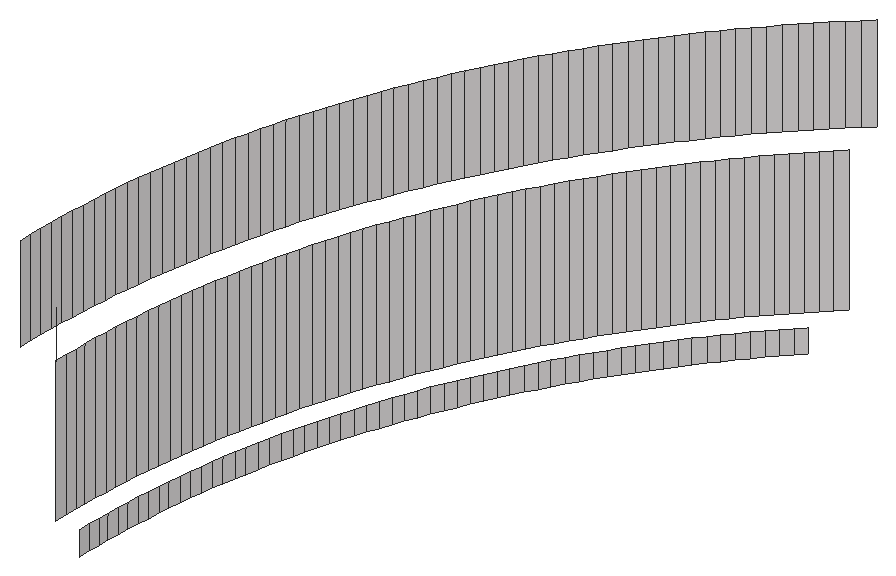
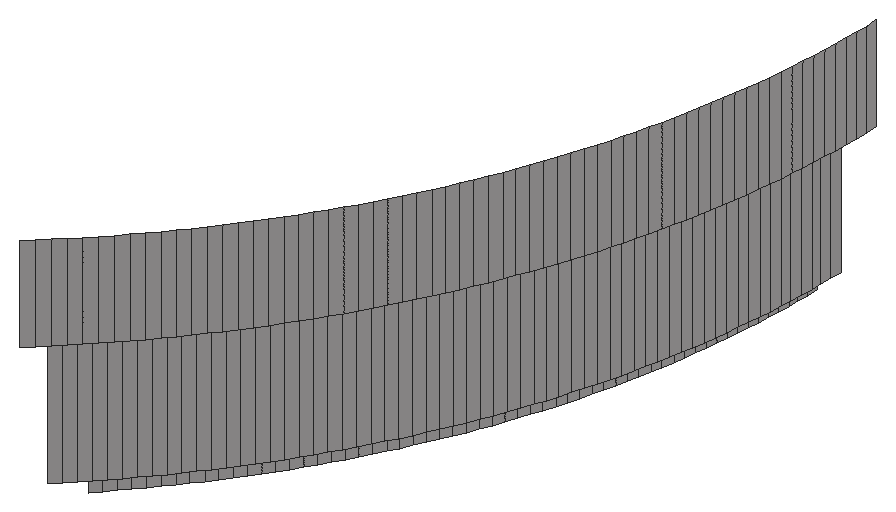
# SketchUp Ruby script. Lengths in inches.
U = 1.inch
M = Sketchup.active_model
def pt(a) = Geom::Point3d.new(a.map { |v| v * U })
def face(e, loops, mat)
  f = e.add_face(loops[0].map { |a| pt(a) })
  loops[1..].each { |l| e.add_face(l.map { |a| pt(a) }).erase! }
  f.material = f.back_material = mat if mat
  f
end
# faces: each face lists its corners as indices into pts; further lists are holes
def faces(e, pts, list, mat = nil) = list.each { |f| face(e, (f[0].is_a?(Array) ? f : [f]).map { |l| l.map { |i| pts[i] } }, mat) }
# xy, xz, yz: faces in a plane at the given z, y or x. An outline is a flat list of corners, or four numbers for a rectangle; further outlines are holes
def ring(l) = l.size == 4 ? [[l[0], l[1]], [l[2], l[1]], [l[2], l[3]], [l[0], l[3]]] : l.each_slice(2).to_a
def flat(e, list, mat, &to3) = list.each { |f| face(e, (f[0].is_a?(Array) ? f : [f]).map { |l| ring(l).map { |u, v| to3.(u, v) } }, mat) }
def xy(e, z, list, mat = nil) = flat(e, list, mat) { |x, y| [x, y, z] }
def xz(e, y, list, mat = nil) = flat(e, list, mat) { |x, z| [x, y, z] }
def yz(e, x, list, mat = nil) = flat(e, list, mat) { |y, z| [x, y, z] }
def lines(e, pts, list) = list.each { |a, b| e.add_line(pt(pts[a]), pt(pts[b])) }
# prism: a flat outline (further loops are holes) pulled along v
def prism(e, loops, v, mat = nil)
  f = face(e, loops, mat); d = Geom::Vector3d.new(v.map { |x| x * U })
  f.pushpull(f.normal.samedirection?(d) ? d.length : -d.length)
end
def box(e, o, s, mat = nil) = prism(e, [[o, [o[0] + s[0], o[1], o[2]], [o[0] + s[0], o[1] + s[1], o[2]], [o[0], o[1] + s[1], o[2]]]], [0, 0, s[2]], mat)
def at(x, y, z, deg = 0) = Geom::Transformation.translation(pt([x, y, z])) * Geom::Transformation.rotation(ORIGIN, Z_AXIS, deg.degrees)
def axes(o, x, y, z) = Geom::Transformation.new([*x, 0, *y, 0, *z, 0, *pt(o).to_a, 1])
def part(name) = M.definitions.add(name)
# library, detail: a bought-in or finely detailed component or shape, given as its bounding box
def library(name, o, s) = part(name).tap { |d| box(d.entities, o, s) }
def detail(e, o, s) = box(e.add_group.entities, o, s)
def put(e, d, t, mat = nil) = e.add_instance(d, t).tap { |i| i.material = mat if mat }
def group(e, t, mat = nil) = e.add_group.tap { |g| g.transformation = t; g.material = mat if mat }.entities
root = M.entities
M.materials.add("[Quartz Light Brown]").color = [215, 212, 212]
yz(root,185.5,[[440.7,493,441.22,497]],"[Quartz Light Brown]")
yz(root,187,[[440.7,487,441.2,493]],"[Quartz Light Brown]")
yz(root,188,[[440.7,486,441.19,487]],"[Quartz Light Brown]")
p = [[188.01,441.67,486],[188,441.19,486],[188,441.19,487],[188.01,441.67,487],[188.03,442.15,486],[188.03,442.15,487],
  [188.05,442.64,486],[188.05,442.64,487],[188.08,443.12,486],[188.08,443.12,487],[188.11,443.6,486],[188.11,443.6,487],
  [188.16,444.09,486],[188.16,444.09,487],[188.2,444.57,486],[188.2,444.57,487],[188.26,445.05,486],[188.26,445.05,487],
  [188.32,445.53,486],[188.32,445.53,487],[188.38,446.01,486],[188.38,446.01,487],[188.46,446.49,486],[188.46,446.49,487],
  [188.53,446.97,486],[188.53,446.97,487],[188.62,447.44,486],[188.62,447.44,487],[188.71,447.92,486],[188.71,447.92,487],
  [188.81,448.39,486],[188.81,448.39,487],[188.91,448.87,486],[188.91,448.87,487],[189.02,449.34,486],[189.02,449.34,487],
  [189.14,449.81,486],[189.14,449.81,487],[189.26,450.28,486],[189.26,450.28,487],[189.39,450.74,486],[189.39,450.74,487],
  [189.52,451.21,486],[189.52,451.21,487],[189.66,451.67,486],[189.66,451.67,487],[189.8125,452.13,486],[189.8125,452.13,487],
  [189.96,452.59,486],[189.96,452.59,487],[190.12,453.05,486],[190.12,453.05,487],[190.29,453.51,486],[190.29,453.51,487],
  [190.46,453.96,486],[190.46,453.96,487],[190.63,454.41,486],[190.63,454.41,487],[190.82,454.86,486],[190.82,454.86,487],
  [191,455.31,486],[191,455.31,487],[191.2,455.75,486],[191.2,455.75,487],[191.4,456.19,486],[191.4,456.19,487],
  [191.6,456.63,486],[191.6,456.63,487],[191.82,457.07,486],[191.82,457.07,487],[192.03,457.5,486],[192.03,457.5,487],
  [192.26,457.93,486],[192.26,457.93,487],[192.48,458.36,486],[192.48,458.36,487],[192.72,458.78,486],[192.72,458.78,487],
  [192.96,459.2,486],[192.96,459.2,487],[193.2,459.62,486],[193.2,459.62,487],[193.45,460.03,486],[193.45,460.03,487],
  [193.71,460.44,486],[193.71,460.44,487],[193.97,460.85,486],[193.97,460.85,487],[194.24,461.26,486],[194.24,461.26,487],
  [194.51,461.66,486],[194.51,461.66,487],[194.78,462.06,486],[194.78,462.06,487],[195.07,462.45,486],[195.07,462.45,487],
  [195.35,462.84,486],[195.35,462.84,487],[195.65,463.23,486],[195.65,463.23,487],[195.94,463.61,486],[195.94,463.61,487],
  [196.25,463.99,486],[196.25,463.99,487],[196.55,464.36,486],[196.55,464.36,487],[196.86,464.73,486],[196.86,464.73,487],
  [197.18,465.1,486],[197.18,465.1,487],[197.5,465.46,486],[197.5,465.46,487],[197.83,465.82,486],[197.83,465.82,487],
  [198.16,466.17,486],[198.16,466.17,487],[187,441.2,487],[187,441.2,493],[187.01,441.7,493],[187.01,441.7,487],
  [187.03,442.19,493],[187.03,442.19,487],[187.05,442.69,493],[187.05,442.69,487],[187.08,443.1875,493],[187.08,443.1875,487],
  [187.12,443.68,493],[187.12,443.68,487],[187.16,444.18,493],[187.16,444.18,487],[187.21,444.67,493],[187.21,444.67,487],
  [187.26,445.17,493],[187.26,445.17,487],[187.33,445.66,493],[187.33,445.66,487],[187.39,446.15,493],[187.39,446.15,487],
  [187.47,446.65,493],[187.47,446.65,487],[187.55,447.14,493],[187.55,447.14,487],[187.64,447.625,493],[187.64,447.625,487],
  [187.73,448.11,493],[187.73,448.11,487],[187.83,448.6,493],[187.83,448.6,487],[187.9375,449.09,493],[187.9375,449.09,487],
  [188.05,449.57,493],[188.05,449.57,487],[188.17,450.05,493],[188.17,450.05,487],[188.29,450.54,493],[188.29,450.54,487],
  [188.43,451.02,493],[188.43,451.02,487],[188.56,451.49,493],[188.56,451.49,487],[188.71,451.97,493],[188.71,451.97,487],
  [188.86,452.44,493],[188.86,452.44,487],[189.02,452.92,493],[189.02,452.92,487],[189.18,453.39,493],[189.18,453.39,487],
  [189.35,453.85,493],[189.35,453.85,487],[189.52,454.32,493],[189.52,454.32,487],[189.71,454.78,493],[189.71,454.78,487],
  [189.89,455.24,493],[189.89,455.24,487],[190.09,455.7,493],[190.09,455.7,487],[190.29,456.16,493],[190.29,456.16,487],
  [190.49,456.61,493],[190.49,456.61,487],[190.7,457.06,493],[190.7,457.06,487],[190.92,457.51,493],[190.92,457.51,487],
  [191.14,457.95,493],[191.14,457.95,487],[191.37,458.39,493],[191.37,458.39,487],[191.6,458.83,493],[191.6,458.83,487],
  [191.85,459.27,493],[191.85,459.27,487],[192.09,459.7,493],[192.09,459.7,487],[192.34,460.13,493],[192.34,460.13,487],
  [192.6,460.56,493],[192.6,460.56,487],[192.86,460.98,493],[192.86,460.98,487],[193.13,461.4,493],[193.13,461.4,487],
  [193.4,461.8125,493],[193.4,461.8125,487],[193.68,462.22,493],[193.68,462.22,487],[193.97,462.63,493],[193.97,462.63,487],
  [194.26,463.04,493],[194.26,463.04,487],[194.55,463.4375,493],[194.55,463.4375,487],[194.85,463.83,493],[194.85,463.83,487],
  [195.16,464.23,493],[195.16,464.23,487],[195.47,464.62,493],[195.47,464.62,487],[195.78,465,493],[195.78,465,487],
  [196.1,465.38,493],[196.1,465.38,487],[196.43,465.76,493],[196.43,465.76,487],[196.76,466.13,493],[196.76,466.13,487],
  [197.1,466.5,493],[197.1,466.5,487],[197.4375,466.86,493],[197.4375,466.86,487],[197.78,467.22,493],[197.78,467.22,487],
  [198.13,467.57,493],[198.13,467.57,487],[198.48,467.92,493],[198.48,467.92,487],[185.51,441.73,493],[185.5,441.22,493],
  [185.5,441.22,497],[185.51,441.73,497],[185.53,442.25,493],[185.53,442.25,497],[185.55,442.77,493],[185.55,442.77,497],
  [185.58,443.28,493],[185.58,443.28,497],[185.62,443.8,493],[185.62,443.8,497],[185.67,444.32,493],[185.67,444.32,497],
  [185.72,444.83,493],[185.72,444.83,497],[185.77,445.34,493],[185.77,445.34,497],[185.84,445.86,493],[185.84,445.86,497],
  [185.91,446.37,493],[185.91,446.37,497],[185.99,446.88,493],[185.99,446.88,497],[186.07,447.39,493],[186.07,447.39,497],
  [186.16,447.9,493],[186.16,447.9,497],[186.26,448.41,493],[186.26,448.41,497],[186.36,448.91,493],[186.36,448.91,497],
  [186.47,449.42,493],[186.47,449.42,497],[186.59,449.92,493],[186.59,449.92,497],[186.72,450.42,493],[186.72,450.42,497],
  [186.85,450.92,493],[186.85,450.92,497],[186.98,451.42,493],[186.98,451.42,497],[187.125,451.92,493],[187.125,451.92,497],
  [187.28,452.41,493],[187.28,452.41,497],[187.43,452.91,493],[187.43,452.91,497],[187.6,453.4,493],[187.6,453.4,497],
  [187.77,453.89,493],[187.77,453.89,497],[187.94,454.37,493],[187.94,454.37,497],[188.125,454.86,493],[188.125,454.86,497],
  [188.3125,455.34,493],[188.3125,455.34,497],[188.51,455.82,493],[188.51,455.82,497],[188.71,456.29,493],[188.71,456.29,497],
  [188.91,456.77,493],[188.91,456.77,497],[189.13,457.24,493],[189.13,457.24,497],[189.35,457.71,493],[189.35,457.71,497],
  [189.57,458.17,493],[189.57,458.17,497],[189.81,458.63,493],[189.81,458.63,497],[190.04,459.09,493],[190.04,459.09,497],
  [190.29,459.55,493],[190.29,459.55,497],[190.54,460,493],[190.54,460,497],[190.79,460.45,493],[190.79,460.45,497],
  [191.05,460.9,493],[191.05,460.9,497],[191.32,461.34,493],[191.32,461.34,497],[191.59,461.78,493],[191.59,461.78,497],
  [191.87,462.21,493],[191.87,462.21,497],[192.16,462.65,493],[192.16,462.65,497],[192.45,463.07,493],[192.45,463.07,497],
  [192.74,463.5,493],[192.74,463.5,497],[193.04,463.92,493],[193.04,463.92,497],[193.35,464.33,493],[193.35,464.33,497],
  [193.66,464.75,493],[193.66,464.75,497],[193.98,465.16,493],[193.98,465.16,497],[194.3,465.56,493],[194.3,465.56,497],
  [194.63,465.96,493],[194.63,465.96,497],[194.96,466.35,493],[194.96,466.35,497],[195.3,466.75,493],[195.3,466.75,497],
  [195.65,467.13,493],[195.65,467.13,497],[195.99,467.51,493],[195.99,467.51,497],[196.35,467.89,493],[196.35,467.89,497],
  [196.71,468.26,493],[196.71,468.26,497],[197.07,468.63,493],[197.07,468.63,497],[197.4375,468.99,493],[197.4375,468.99,497],
  [197.81,469.35,493],[197.81,469.35,497],[198.1875,469.71,493],[198.1875,469.71,497],[187,440.7,493],[187,440.7,495]]
faces(root,p,[[0,1,2,3],[4,0,3,5],[6,4,5,7],[8,6,7,9],[10,8,9,11],[12,10,11,13],[14,12,13,15],[16,14,15,17],
  [18,16,17,19],[20,18,19,21],[22,20,21,23],[24,22,23,25],[26,24,25,27],[28,26,27,29],[30,28,29,31],[32,30,31,33],
  [34,32,33,35],[36,34,35,37],[38,36,37,39],[40,38,39,41],[42,40,41,43],[44,42,43,45],[46,44,45,47],[48,46,47,49],
  [50,48,49,51],[52,50,51,53],[54,52,53,55],[56,54,55,57],[58,56,57,59],[60,58,59,61],[62,60,61,63],[64,62,63,65],
  [66,64,65,67],[68,66,67,69],[70,68,69,71],[72,70,71,73],[74,72,73,75],[76,74,75,77],[78,76,77,79],[80,78,79,81],
  [82,80,81,83],[84,82,83,85],[86,84,85,87],[88,86,87,89],[90,88,89,91],[92,90,91,93],[94,92,93,95],[96,94,95,97],
  [98,96,97,99],[100,98,99,101],[102,100,101,103],[104,102,103,105],[106,104,105,107],[108,106,107,109],[110,108,109,111],[112,110,111,113],
  [114,112,113,115],[116,117,118,119],[119,118,120,121],[121,120,122,123],[123,122,124,125],[125,124,126,127],[127,126,128,129],[129,128,130,131],
  [131,130,132,133],[133,132,134,135],[135,134,136,137],[137,136,138,139],[139,138,140,141],[141,140,142,143],[143,142,144,145],[145,144,146,147],
  [147,146,148,149],[149,148,150,151],[151,150,152,153],[153,152,154,155],[155,154,156,157],[157,156,158,159],[159,158,160,161],[161,160,162,163],
  [163,162,164,165],[165,164,166,167],[167,166,168,169],[169,168,170,171],[171,170,172,173],[173,172,174,175],[175,174,176,177],[177,176,178,179],
  [179,178,180,181],[181,180,182,183],[183,182,184,185],[185,184,186,187],[187,186,188,189],[189,188,190,191],[191,190,192,193],[193,192,194,195],
  [195,194,196,197],[197,196,198,199],[199,198,200,201],[201,200,202,203],[203,202,204,205],[205,204,206,207],[207,206,208,209],[209,208,210,211],
  [211,210,212,213],[213,212,214,215],[215,214,216,217],[217,216,218,219],[219,218,220,221],[221,220,222,223],[223,222,224,225],[225,224,226,227],
  [227,226,228,229],[229,228,230,231],[231,230,232,233],[233,232,234,235],[235,234,236,237],[238,239,240,241],[242,238,241,243],[244,242,243,245],
  [246,244,245,247],[248,246,247,249],[250,248,249,251],[252,250,251,253],[254,252,253,255],[256,254,255,257],[258,256,257,259],[260,258,259,261],
  [262,260,261,263],[264,262,263,265],[266,264,265,267],[268,266,267,269],[270,268,269,271],[272,270,271,273],[274,272,273,275],[276,274,275,277],
  [278,276,277,279],[280,278,279,281],[282,280,281,283],[284,282,283,285],[286,284,285,287],[288,286,287,289],[290,288,289,291],[292,290,291,293],
  [294,292,293,295],[296,294,295,297],[298,296,297,299],[300,298,299,301],[302,300,301,303],[304,302,303,305],[306,304,305,307],[308,306,307,309],
  [310,308,309,311],[312,310,311,313],[314,312,313,315],[316,314,315,317],[318,316,317,319],[320,318,319,321],[322,320,321,323],[324,322,323,325],
  [326,324,325,327],[328,326,327,329],[330,328,329,331],[332,330,331,333],[334,332,333,335],[336,334,335,337],[338,336,337,339],[340,338,339,341],
  [342,340,341,343],[344,342,343,345],[346,344,345,347],[348,346,347,349],[350,348,349,351],[352,350,351,353],[354,352,353,355],[356,354,355,357],
  [358,356,357,359],[360,358,359,361],[362,360,361,363]],"[Quartz Light Brown]")
lines(root,p,[[364,365]])
